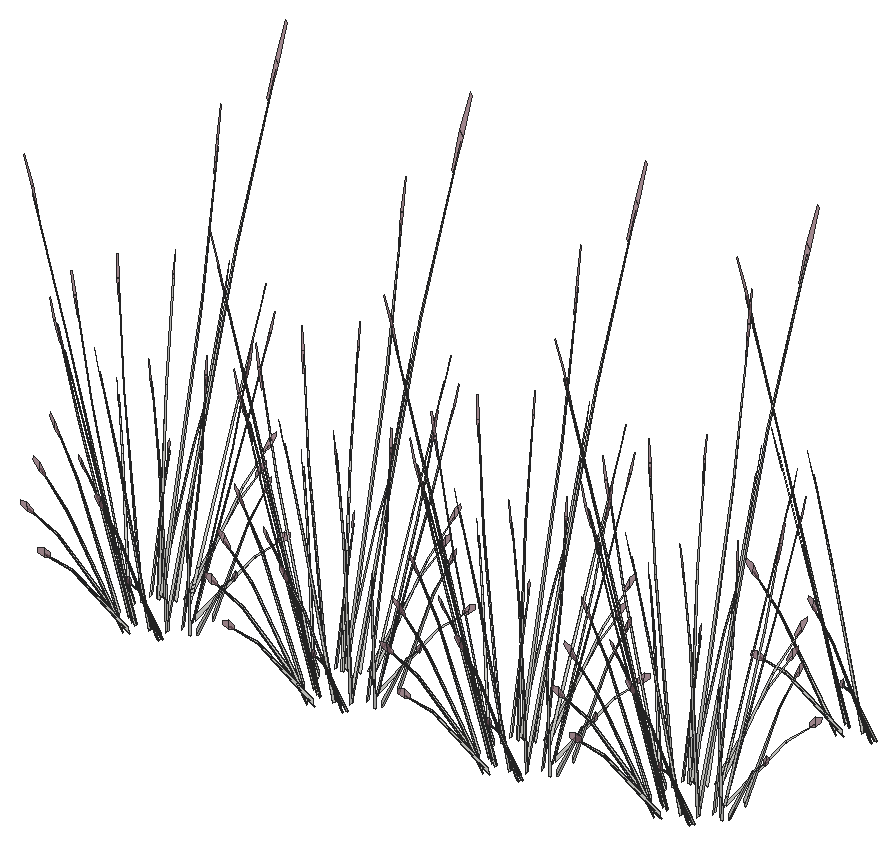
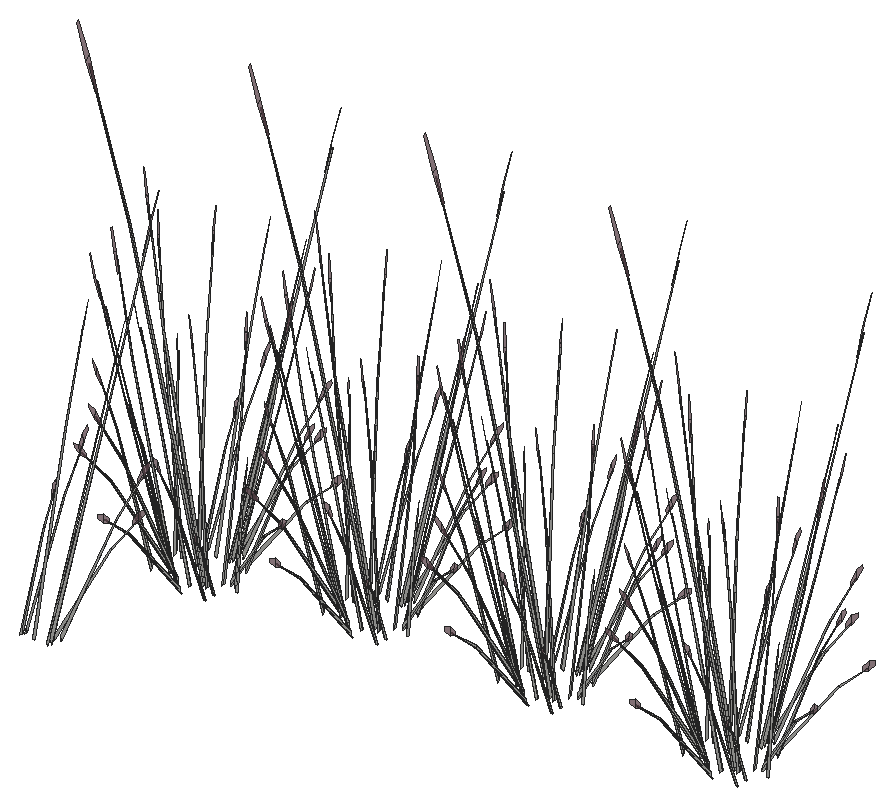
# SketchUp Ruby script. Lengths in inches.
U = 1.inch
M = Sketchup.active_model
def pt(a) = Geom::Point3d.new(a.map { |v| v * U })
def face(e, loops, mat)
  f = e.add_face(loops[0].map { |a| pt(a) })
  loops[1..].each { |l| e.add_face(l.map { |a| pt(a) }).erase! }
  f.material = f.back_material = mat if mat
  f
end
# faces: each face lists its corners as indices into pts; further lists are holes
def faces(e, pts, list, mat = nil) = list.each { |f| face(e, (f[0].is_a?(Array) ? f : [f]).map { |l| l.map { |i| pts[i] } }, mat) }
# xy, xz, yz: faces in a plane at the given z, y or x. An outline is a flat list of corners, or four numbers for a rectangle; further outlines are holes
def ring(l) = l.size == 4 ? [[l[0], l[1]], [l[2], l[1]], [l[2], l[3]], [l[0], l[3]]] : l.each_slice(2).to_a
def flat(e, list, mat, &to3) = list.each { |f| face(e, (f[0].is_a?(Array) ? f : [f]).map { |l| ring(l).map { |u, v| to3.(u, v) } }, mat) }
def xy(e, z, list, mat = nil) = flat(e, list, mat) { |x, y| [x, y, z] }
def xz(e, y, list, mat = nil) = flat(e, list, mat) { |x, z| [x, y, z] }
def yz(e, x, list, mat = nil) = flat(e, list, mat) { |y, z| [x, y, z] }
def lines(e, pts, list) = list.each { |a, b| e.add_line(pt(pts[a]), pt(pts[b])) }
# prism: a flat outline (further loops are holes) pulled along v
def prism(e, loops, v, mat = nil)
  f = face(e, loops, mat); d = Geom::Vector3d.new(v.map { |x| x * U })
  f.pushpull(f.normal.samedirection?(d) ? d.length : -d.length)
end
def box(e, o, s, mat = nil) = prism(e, [[o, [o[0] + s[0], o[1], o[2]], [o[0] + s[0], o[1] + s[1], o[2]], [o[0], o[1] + s[1], o[2]]]], [0, 0, s[2]], mat)
def at(x, y, z, deg = 0) = Geom::Transformation.translation(pt([x, y, z])) * Geom::Transformation.rotation(ORIGIN, Z_AXIS, deg.degrees)
def axes(o, x, y, z) = Geom::Transformation.new([*x, 0, *y, 0, *z, 0, *pt(o).to_a, 1])
def part(name) = M.definitions.add(name)
# library, detail: a bought-in or finely detailed component or shape, given as its bounding box
def library(name, o, s) = part(name).tap { |d| box(d.entities, o, s) }
def detail(e, o, s) = box(e.add_group.entities, o, s)
def put(e, d, t, mat = nil) = e.add_instance(d, t).tap { |i| i.material = mat if mat }
def group(e, t, mat = nil) = e.add_group.tap { |g| g.transformation = t; g.material = mat if mat }.entities
root = M.entities
M.materials.add("LightPink_Translucent").color = [144, 107, 117]
M.materials["LightPink_Translucent"].alpha = 0.75
c1 = part("blade")
p = [[2.15,0.21,22],[0,0.17,0],[0.09,0.45,0],[2.18,0.31,22],[2.29,0.31,22],[0.38,0.45,0],
  [2.48,0.24,33],[2.49,0.24,33],[2.48,0.22,33]]
faces(c1.entities,p,[[0,1,2,3],[4,5,2,3],[6,3,4,7],[8,0,3,6]])
c2 = part("seeds")
p = [[0.3,-0.1,1.38],[-0.01,-0.03,1.59],[-0.01,-0.03,0.03],[0.14,-0.07,-0.07],[0.29,-0.03,3],[0.15,0.01,3.11]]
faces(c2.entities,p,[[0,1,2,3],[1,0,4,5]],"LightPink_Translucent")
c3 = part("blade with seeds")
put(c3.entities,c1,at(0,0,0))
put(c3.entities,c2,axes([2.4,0.25,30.99],[1.5799,-0.05474,1.17369],[-0.12525,1.92788,0.29478],[-0.07173,-0.02425,1.56792]))
put(root,c3,axes([318.89,53.77,268.39],[-0.07822,-0.07621,1.62908],[-0.52201,0.04832,-0.25764],[-0.08331,-0.18228,0.13065]))
put(root,c3,axes([302.52,53.77,268.39],[-0.07822,-0.07621,1.62908],[-0.52201,0.04832,-0.25764],[-0.08331,-0.18228,0.13065]))
put(root,c3,axes([285.3,53.77,268.39],[-0.07822,-0.07621,1.62908],[-0.52201,0.04832,-0.25764],[-0.08331,-0.18228,0.13065]))
put(root,c3,axes([321.23,54.7,268.39],[-0.00494,-0.10818,1.62908],[-0.41695,-0.31265,-0.25764],[0.06446,-0.18952,0.13065]))
put(root,c3,axes([304.87,54.7,268.39],[-0.00494,-0.10818,1.62908],[-0.41695,-0.31265,-0.25764],[0.06446,-0.18952,0.13065]))
put(root,c3,axes([287.65,54.7,268.39],[-0.00494,-0.10818,1.62908],[-0.41695,-0.31265,-0.25764],[0.06446,-0.18952,0.13065]))
put(root,c3,axes([321.12,54.32,268.38],[-0.05194,0.04152,1.65179],[-0.50886,-0.14007,-0.15608],[-0.01842,-0.18118,0.29231]))
put(root,c3,axes([304.76,54.32,268.38],[-0.05194,0.04152,1.65179],[-0.50886,-0.14007,-0.15608],[-0.01842,-0.18118,0.29231]))
put(root,c3,axes([287.54,54.32,268.38],[-0.05194,0.04152,1.65179],[-0.50886,-0.14007,-0.15608],[-0.01842,-0.18118,0.29231]))
put(root,c3,axes([318.35,53.52,268.38],[-0.00954,0.06515,1.65179],[-0.47055,0.23645,-0.15608],[-0.13847,-0.12087,0.29231]))
put(root,c3,axes([301.99,53.52,268.38],[-0.00954,0.06515,1.65179],[-0.47055,0.23645,-0.15608],[-0.13847,-0.12087,0.29231]))
put(root,c3,axes([284.77,53.52,268.38],[-0.00954,0.06515,1.65179],[-0.47055,0.23645,-0.15608],[-0.13847,-0.12087,0.29231]))
put(root,c3,axes([319.67,54.74,268.4],[0.37684,-0.18473,0.05988],[0.18445,0.33686,0.47138],[-0.03639,-0.14849,0.71878]))
put(root,c3,axes([303.31,54.74,268.4],[0.37684,-0.18473,0.05988],[0.18445,0.33686,0.47138],[-0.03639,-0.14849,0.71878]))
put(root,c3,axes([286.09,54.74,268.4],[0.37684,-0.18473,0.05988],[0.18445,0.33686,0.47138],[-0.03639,-0.14849,0.71878]))
put(root,c3,axes([318.38,54.79,268.4],[0.23243,-0.34529,0.05988],[0.331,0.20103,0.47138],[-0.10701,-0.1107,0.71878]))
put(root,c3,axes([302.01,54.79,268.4],[0.23243,-0.34529,0.05988],[0.331,0.20103,0.47138],[-0.10701,-0.1107,0.71878]))
put(root,c3,axes([284.79,54.79,268.4],[0.23243,-0.34529,0.05988],[0.331,0.20103,0.47138],[-0.10701,-0.1107,0.71878]))
put(root,c3,axes([318.48,54.76,269.06],[-0.34131,0.52108,-0.12682],[-0.49429,-0.3002,-0.70393],[-0.17182,-0.14722,1.06961]))
put(root,c3,axes([302.12,54.76,269.06],[-0.34131,0.52108,-0.12682],[-0.49429,-0.3002,-0.70393],[-0.17182,-0.14722,1.06961]))
put(root,c3,axes([284.9,54.76,269.06],[-0.34131,0.52108,-0.12682],[-0.49429,-0.3002,-0.70393],[-0.17182,-0.14722,1.06961]))
put(root,c3,axes([320.8125,55.33,268.4],[0.42027,0.02533,0.05988],[-0.01152,0.38243,0.47138],[0.04398,-0.14649,0.71878]))
put(root,c3,axes([304.45,55.33,268.4],[0.42027,0.02533,0.05988],[-0.01152,0.38243,0.47138],[0.04398,-0.14649,0.71878]))
put(root,c3,axes([287.23,55.33,268.4],[0.42027,0.02533,0.05988],[-0.01152,0.38243,0.47138],[0.04398,-0.14649,0.71878]))
put(root,c3,axes([332.72,56.47,268.39],[-0.07822,-0.07621,1.62908],[-0.52201,0.04832,-0.25764],[-0.08331,-0.18228,0.13065]))
put(root,c3,axes([317.17,54.61,268.39],[-0.11004,-0.00384,1.62908],[-0.35032,0.38367,-0.25764],[-0.18692,-0.07839,0.13065]))
put(root,c3,axes([300.81,54.61,268.39],[-0.11004,-0.00384,1.62908],[-0.35032,0.38367,-0.25764],[-0.18692,-0.07839,0.13065]))
put(root,c3,axes([283.59,54.61,268.39],[-0.11004,-0.00384,1.62908],[-0.35032,0.38367,-0.25764],[-0.18692,-0.07839,0.13065]))
put(root,c3,axes([322.5,56.39,268.38],[-0.0668,-0.00413,1.65179],[-0.27738,-0.44233,-0.15608],[0.11139,-0.14544,0.29231]))
put(root,c3,axes([306.13,56.39,268.38],[-0.0668,-0.00413,1.65179],[-0.27738,-0.44233,-0.15608],[0.11139,-0.14544,0.29231]))
put(root,c3,axes([288.91,56.39,268.38],[-0.0668,-0.00413,1.65179],[-0.27738,-0.44233,-0.15608],[0.11139,-0.14544,0.29231]))
put(root,c3,axes([335.0625,57.4,268.39],[-0.00494,-0.10818,1.62908],[-0.41695,-0.31265,-0.25764],[0.06446,-0.18952,0.13065]))
put(root,c3,axes([334.95,57.01,268.38],[-0.05194,0.04152,1.65179],[-0.50886,-0.14007,-0.15608],[-0.01842,-0.18118,0.29231]))
put(root,c3,axes([317.29,55.47,268.4],[0.02575,-0.41332,0.05988],[0.38885,0.01133,0.47138],[-0.14895,-0.04325,0.71878]))
put(root,c3,axes([300.92,55.47,268.4],[0.02575,-0.41332,0.05988],[0.38885,0.01133,0.47138],[-0.14895,-0.04325,0.71878]))
put(root,c3,axes([283.7,55.47,268.4],[0.02575,-0.41332,0.05988],[0.38885,0.01133,0.47138],[-0.14895,-0.04325,0.71878]))
put(root,c3,axes([332.18,56.22,268.38],[-0.00954,0.06515,1.65179],[-0.47055,0.23645,-0.15608],[-0.13847,-0.12087,0.29231]))
put(root,c3,axes([333.5,57.44,268.4],[0.37684,-0.18473,0.05988],[0.18445,0.33686,0.47138],[-0.03639,-0.14849,0.71878]))
put(root,c3,axes([321.5,56.41,268.4],[0.35109,0.22859,0.05988],[-0.2044,0.32553,0.47138],[0.11256,-0.10524,0.71878]))
put(root,c3,axes([305.14,56.41,268.4],[0.35109,0.22859,0.05988],[-0.2044,0.32553,0.47138],[0.11256,-0.10524,0.71878]))
put(root,c3,axes([287.92,56.41,268.4],[0.35109,0.22859,0.05988],[-0.2044,0.32553,0.47138],[0.11256,-0.10524,0.71878]))
put(root,c3,axes([322.75,56.92,268.39],[0.07097,-0.08279,1.62908],[-0.09083,-0.50786,-0.25764],[0.17806,-0.09629,0.13065]))
put(root,c3,axes([306.38,56.92,268.39],[0.07097,-0.08279,1.62908],[-0.09083,-0.50786,-0.25764],[0.17806,-0.09629,0.13065]))
put(root,c3,axes([289.16,56.92,268.39],[0.07097,-0.08279,1.62908],[-0.09083,-0.50786,-0.25764],[0.17806,-0.09629,0.13065]))
put(root,c3,axes([332.21,57.49,268.4],[0.23243,-0.34529,0.05988],[0.331,0.20103,0.47138],[-0.10701,-0.1107,0.71878]))
put(root,c3,axes([316.75,54.93,268.38],[0.03791,0.05424,1.65179],[-0.18278,0.48761,-0.15608],[-0.18511,0.00353,0.29231]))
put(root,c3,axes([300.39,54.93,268.38],[0.03791,0.05424,1.65179],[-0.18278,0.48761,-0.15608],[-0.18511,0.00353,0.29231]))
put(root,c3,axes([283.17,54.93,268.38],[0.03791,0.05424,1.65179],[-0.18278,0.48761,-0.15608],[-0.18511,0.00353,0.29231]))
put(root,c3,axes([332.3125,57.46,269.06],[-0.34131,0.52108,-0.12682],[-0.49429,-0.3002,-0.70393],[-0.17182,-0.14722,1.06961]))
put(root,c3,axes([334.65,58.03,268.4],[0.42027,0.02533,0.05988],[-0.01152,0.38243,0.47138],[0.04398,-0.14649,0.71878]))
put(root,c3,axes([331.01,57.31,268.39],[-0.11004,-0.00384,1.62908],[-0.35032,0.38367,-0.25764],[-0.18692,-0.07839,0.13065]))
put(root,c3,axes([336.33,59.08,268.38],[-0.0668,-0.00413,1.65179],[-0.27738,-0.44233,-0.15608],[0.11139,-0.14544,0.29231]))
put(root,c3,axes([316.6875,56.6,268.4],[-0.18783,-0.37061,0.05988],[0.34252,-0.1814,0.47138],[-0.15099,0.03579,0.71878]))
put(root,c3,axes([300.32,56.6,268.4],[-0.18783,-0.37061,0.05988],[0.34252,-0.1814,0.47138],[-0.15099,0.03579,0.71878]))
put(root,c3,axes([283.1,56.6,268.4],[-0.18783,-0.37061,0.05988],[0.34252,-0.1814,0.47138],[-0.15099,0.03579,0.71878]))
put(root,c3,axes([331.12,58.17,268.4],[0.02575,-0.41332,0.05988],[0.38885,0.01133,0.47138],[-0.14895,-0.04325,0.71878]))
put(root,c3,axes([335.34,59.1,268.4],[0.35109,0.22859,0.05988],[-0.2044,0.32553,0.47138],[0.11256,-0.10524,0.71878]))
put(root,c3,axes([321.56,57.68,268.4],[0.18783,0.37061,0.05988],[-0.34252,0.1814,0.47138],[0.15099,-0.03579,0.71878]))
put(root,c3,axes([305.19,57.68,268.4],[0.18783,0.37061,0.05988],[-0.34252,0.1814,0.47138],[0.15099,-0.03579,0.71878]))
put(root,c3,axes([287.97,57.68,268.4],[0.18783,0.37061,0.05988],[-0.34252,0.1814,0.47138],[0.15099,-0.03579,0.71878]))
put(root,c3,axes([336.58,59.61,268.39],[0.07097,-0.08279,1.62908],[-0.09083,-0.50786,-0.25764],[0.17806,-0.09629,0.13065]))
put(root,c3,axes([330.58,57.63,268.38],[0.03791,0.05424,1.65179],[-0.18278,0.48761,-0.15608],[-0.18511,0.00353,0.29231]))
put(root,c3,axes([322.375,59.15,268.38],[-0.04624,-0.04758,1.65179],[0.10116,-0.51007,-0.15608],[0.18215,-0.03259,0.29231]))
put(root,c3,axes([306.01,59.15,268.38],[-0.04624,-0.04758,1.65179],[0.10116,-0.51007,-0.15608],[0.18215,-0.03259,0.29231]))
put(root,c3,axes([288.79,59.15,268.38],[-0.04624,-0.04758,1.65179],[0.10116,-0.51007,-0.15608],[0.18215,-0.03259,0.29231]))
put(root,c3,axes([316.35,57.08,268.39],[-0.08351,0.07057,1.62908],[0.0071,0.51561,-0.25764],[-0.19143,0.06705,0.13065]))
put(root,c3,axes([299.99,57.08,268.39],[-0.08351,0.07057,1.62908],[0.0071,0.51561,-0.25764],[-0.19143,0.06705,0.13065]))
put(root,c3,axes([282.77,57.08,268.39],[-0.08351,0.07057,1.62908],[0.0071,0.51561,-0.25764],[-0.19143,0.06705,0.13065]))
put(root,c3,axes([321.22,58.38,268.39],[0.10971,-0.00919,1.62908],[0.30091,-0.42228,-0.25764],[0.19514,0.05574,0.13065]))
put(root,c3,axes([304.86,58.38,268.39],[0.10971,-0.00919,1.62908],[0.30091,-0.42228,-0.25764],[0.19514,0.05574,0.13065]))
put(root,c3,axes([287.64,58.38,268.39],[0.10971,-0.00919,1.62908],[0.30091,-0.42228,-0.25764],[0.19514,0.05574,0.13065]))
put(root,c3,axes([330.52,59.3,268.4],[-0.18783,-0.37061,0.05988],[0.34252,-0.1814,0.47138],[-0.15099,0.03579,0.71878]))
put(root,c3,axes([316.74,57.87,268.4],[-0.35109,-0.22859,0.05988],[0.2044,-0.32553,0.47138],[-0.11256,0.10524,0.71878]))
put(root,c3,axes([300.375,57.87,268.4],[-0.35109,-0.22859,0.05988],[0.2044,-0.32553,0.47138],[-0.11256,0.10524,0.71878]))
put(root,c3,axes([283.16,57.87,268.4],[-0.35109,-0.22859,0.05988],[0.2044,-0.32553,0.47138],[-0.11256,0.10524,0.71878]))
put(root,c3,axes([315.43,57.6,268.38],[0.06527,0.01458,1.65179],[0.20191,0.48025,-0.15608],[-0.1336,0.12605,0.29231]))
put(root,c3,axes([299.0625,57.6,268.38],[0.06527,0.01458,1.65179],[0.20191,0.48025,-0.15608],[-0.1336,0.12605,0.29231]))
put(root,c3,axes([281.84,57.6,268.38],[0.06527,0.01458,1.65179],[0.20191,0.48025,-0.15608],[-0.1336,0.12605,0.29231]))
put(root,c3,axes([320.96,58.8,268.4],[-0.02575,0.41332,0.05988],[-0.38885,-0.01133,0.47138],[0.14895,0.04325,0.71878]))
put(root,c3,axes([304.59,58.8,268.4],[-0.02575,0.41332,0.05988],[-0.38885,-0.01133,0.47138],[0.14895,0.04325,0.71878]))
put(root,c3,axes([287.375,58.8,268.4],[-0.02575,0.41332,0.05988],[-0.38885,-0.01133,0.47138],[0.14895,0.04325,0.71878]))
put(root,c3,axes([335.39,60.375,268.4],[0.18783,0.37061,0.05988],[-0.34252,0.1814,0.47138],[0.15099,-0.03579,0.71878]))
put(root,c3,axes([320.1,56.57,268.17],[-0.44191,-0.28242,1.28769],[0.46662,-0.43971,0.5556],[0.14258,0.26499,1.24467]))
put(root,c3,axes([303.73,56.57,268.17],[-0.44191,-0.28242,1.28769],[0.46662,-0.43971,0.5556],[0.14258,0.26499,1.24467]))
put(root,c3,axes([286.51,56.57,268.17],[-0.44191,-0.28242,1.28769],[0.46662,-0.43971,0.5556],[0.14258,0.26499,1.24467]))
put(root,c3,axes([336.21,61.85,268.38],[-0.04624,-0.04758,1.65179],[0.10116,-0.51007,-0.15608],[0.18215,-0.03259,0.29231]))
put(root,c3,axes([330.1875,59.78,268.39],[-0.08351,0.07057,1.62908],[0.0071,0.51561,-0.25764],[-0.19143,0.06705,0.13065]))
put(root,c3,axes([319.35,59.7,268.38],[0.00151,-0.06581,1.65179],[0.43826,-0.29033,-0.15608],[0.15223,0.10363,0.29231]))
put(root,c3,axes([302.99,59.7,268.38],[0.00151,-0.06581,1.65179],[0.43826,-0.29033,-0.15608],[0.15223,0.10363,0.29231]))
put(root,c3,axes([285.77,59.7,268.38],[0.00151,-0.06581,1.65179],[0.43826,-0.29033,-0.15608],[0.15223,0.10363,0.29231]))
put(root,c3,axes([317.43,58.94,268.4],[-0.42027,-0.02533,0.05988],[0.01152,-0.38243,0.47138],[-0.04398,0.14649,0.71878]))
put(root,c3,axes([301.07,58.94,268.4],[-0.42027,-0.02533,0.05988],[0.01152,-0.38243,0.47138],[-0.04398,0.14649,0.71878]))
put(root,c3,axes([283.85,58.94,268.4],[-0.42027,-0.02533,0.05988],[0.01152,-0.38243,0.47138],[-0.04398,0.14649,0.71878]))
put(root,c3,axes([319.86,59.48,268.4],[-0.23243,0.34529,0.05988],[-0.331,-0.20103,0.47138],[0.10701,0.1107,0.71878]))
put(root,c3,axes([303.5,59.48,268.4],[-0.23243,0.34529,0.05988],[-0.331,-0.20103,0.47138],[0.10701,0.1107,0.71878]))
put(root,c3,axes([286.28,59.48,268.4],[-0.23243,0.34529,0.05988],[-0.331,-0.20103,0.47138],[0.10701,0.1107,0.71878]))
put(root,c3,axes([335.06,61.08,268.39],[0.10971,-0.00919,1.62908],[0.30091,-0.42228,-0.25764],[0.19514,0.05574,0.13065]))
put(root,c3,axes([330.57,60.57,268.4],[-0.35109,-0.22859,0.05988],[0.2044,-0.32553,0.47138],[-0.11256,0.10524,0.71878]))
put(root,c3,axes([318.57,59.53,268.4],[-0.37684,0.18473,0.05988],[-0.18445,-0.33686,0.47138],[0.03639,0.14849,0.71878]))
put(root,c3,axes([302.21,59.53,268.4],[-0.37684,0.18473,0.05988],[-0.18445,-0.33686,0.47138],[0.03639,0.14849,0.71878]))
put(root,c3,axes([284.99,59.53,268.4],[-0.37684,0.18473,0.05988],[-0.18445,-0.33686,0.47138],[0.03639,0.14849,0.71878]))
put(root,c3,axes([316.37,59,268.39],[-0.01271,0.10756,1.62908],[0.36076,0.37419,-0.25764],[-0.09444,0.17695,0.13065]))
put(root,c3,axes([300.01,59,268.39],[-0.01271,0.10756,1.62908],[0.36076,0.37419,-0.25764],[-0.09444,0.17695,0.13065]))
put(root,c3,axes([282.79,59,268.39],[-0.01271,0.10756,1.62908],[0.36076,0.37419,-0.25764],[-0.09444,0.17695,0.13065]))
put(root,c3,axes([317.52,58.76,269.03],[0.56206,0.02693,-0.12569],[-0.01536,0.50991,-0.69765],[-0.03904,0.19638,1.06006]))
put(root,c3,axes([301.16,58.76,269.03],[0.56206,0.02693,-0.12569],[-0.01536,0.50991,-0.69765],[-0.03904,0.19638,1.06006]))
put(root,c3,axes([283.9375,58.76,269.03],[0.56206,0.02693,-0.12569],[-0.01536,0.50991,-0.69765],[-0.03904,0.19638,1.06006]))
put(root,c3,axes([329.26,60.3,268.38],[0.06527,0.01458,1.65179],[0.20191,0.48025,-0.15608],[-0.1336,0.12605,0.29231]))
put(root,c3,axes([334.79,61.5,268.4],[-0.02575,0.41332,0.05988],[-0.38885,-0.01133,0.47138],[0.14895,0.04325,0.71878]))
put(root,c3,axes([316.33,60.11,268.38],[0.05802,-0.03282,1.65179],[0.47954,0.21828,-0.15608],[-0.01127,0.18175,0.29231]))
put(root,c3,axes([299.96,60.11,268.38],[0.05802,-0.03282,1.65179],[0.47954,0.21828,-0.15608],[-0.01127,0.18175,0.29231]))
put(root,c3,axes([282.75,60.11,268.38],[0.05802,-0.03282,1.65179],[0.47954,0.21828,-0.15608],[-0.01127,0.18175,0.29231]))
put(root,c3,axes([333.93,59.26,268.17],[-0.44191,-0.28242,1.28769],[0.46662,-0.43971,0.5556],[0.14258,0.26499,1.24467]))
put(root,c3,axes([318.44,60.34,268.39],[0.06483,0.08753,1.62908],[0.52315,0.03439,-0.25764],[0.05261,0.19303,0.13065]))
put(root,c3,axes([302.08,60.34,268.39],[0.06483,0.08753,1.62908],[0.52315,0.03439,-0.25764],[0.05261,0.19303,0.13065]))
put(root,c3,axes([284.86,60.34,268.39],[0.06483,0.08753,1.62908],[0.52315,0.03439,-0.25764],[0.05261,0.19303,0.13065]))
put(root,c3,axes([333.18,62.39,268.38],[0.00151,-0.06581,1.65179],[0.43826,-0.29033,-0.15608],[0.15223,0.10363,0.29231]))
put(root,c3,axes([331.26,61.64,268.4],[-0.42027,-0.02533,0.05988],[0.01152,-0.38243,0.47138],[-0.04398,0.14649,0.71878]))
put(root,c3,axes([333.7,62.18,268.4],[-0.23243,0.34529,0.05988],[-0.331,-0.20103,0.47138],[0.10701,0.1107,0.71878]))
put(root,c3,axes([332.41,62.23,268.4],[-0.37684,0.18473,0.05988],[-0.18445,-0.33686,0.47138],[0.03639,0.14849,0.71878]))
put(root,c3,axes([330.2,61.7,268.39],[-0.01271,0.10756,1.62908],[0.36076,0.37419,-0.25764],[-0.09444,0.17695,0.13065]))
put(root,c3,axes([331.35,61.46,269.03],[0.56206,0.02693,-0.12569],[-0.01536,0.50991,-0.69765],[-0.03904,0.19638,1.06006]))
put(root,c3,axes([330.16,62.8,268.38],[0.05802,-0.03282,1.65179],[0.47954,0.21828,-0.15608],[-0.01127,0.18175,0.29231]))
put(root,c3,axes([332.28,63.03,268.39],[0.06483,0.08753,1.62908],[0.52315,0.03439,-0.25764],[0.05261,0.19303,0.13065]))
put(root,c3,axes([335.41,74.32,268.39],[-0.07822,-0.07621,1.62908],[-0.52201,0.04832,-0.25764],[-0.08331,-0.18228,0.13065]))
put(root,c3,axes([337.76,75.25,268.39],[-0.00494,-0.10818,1.62908],[-0.41695,-0.31265,-0.25764],[0.06446,-0.18952,0.13065]))
put(root,c3,axes([337.65,74.86,268.38],[-0.05194,0.04152,1.65179],[-0.50886,-0.14007,-0.15608],[-0.01842,-0.18118,0.29231]))
put(root,c3,axes([334.88,74.07,268.38],[-0.00954,0.06515,1.65179],[-0.47055,0.23645,-0.15608],[-0.13847,-0.12087,0.29231]))
put(root,c3,axes([336.2,75.29,268.4],[0.37684,-0.18473,0.05988],[0.18445,0.33686,0.47138],[-0.03639,-0.14849,0.71878]))
put(root,c3,axes([334.91,75.34,268.4],[0.23243,-0.34529,0.05988],[0.331,0.20103,0.47138],[-0.10701,-0.1107,0.71878]))
put(root,c3,axes([335.01,75.3,269.06],[-0.34131,0.52108,-0.12682],[-0.49429,-0.3002,-0.70393],[-0.17182,-0.14722,1.06961]))
